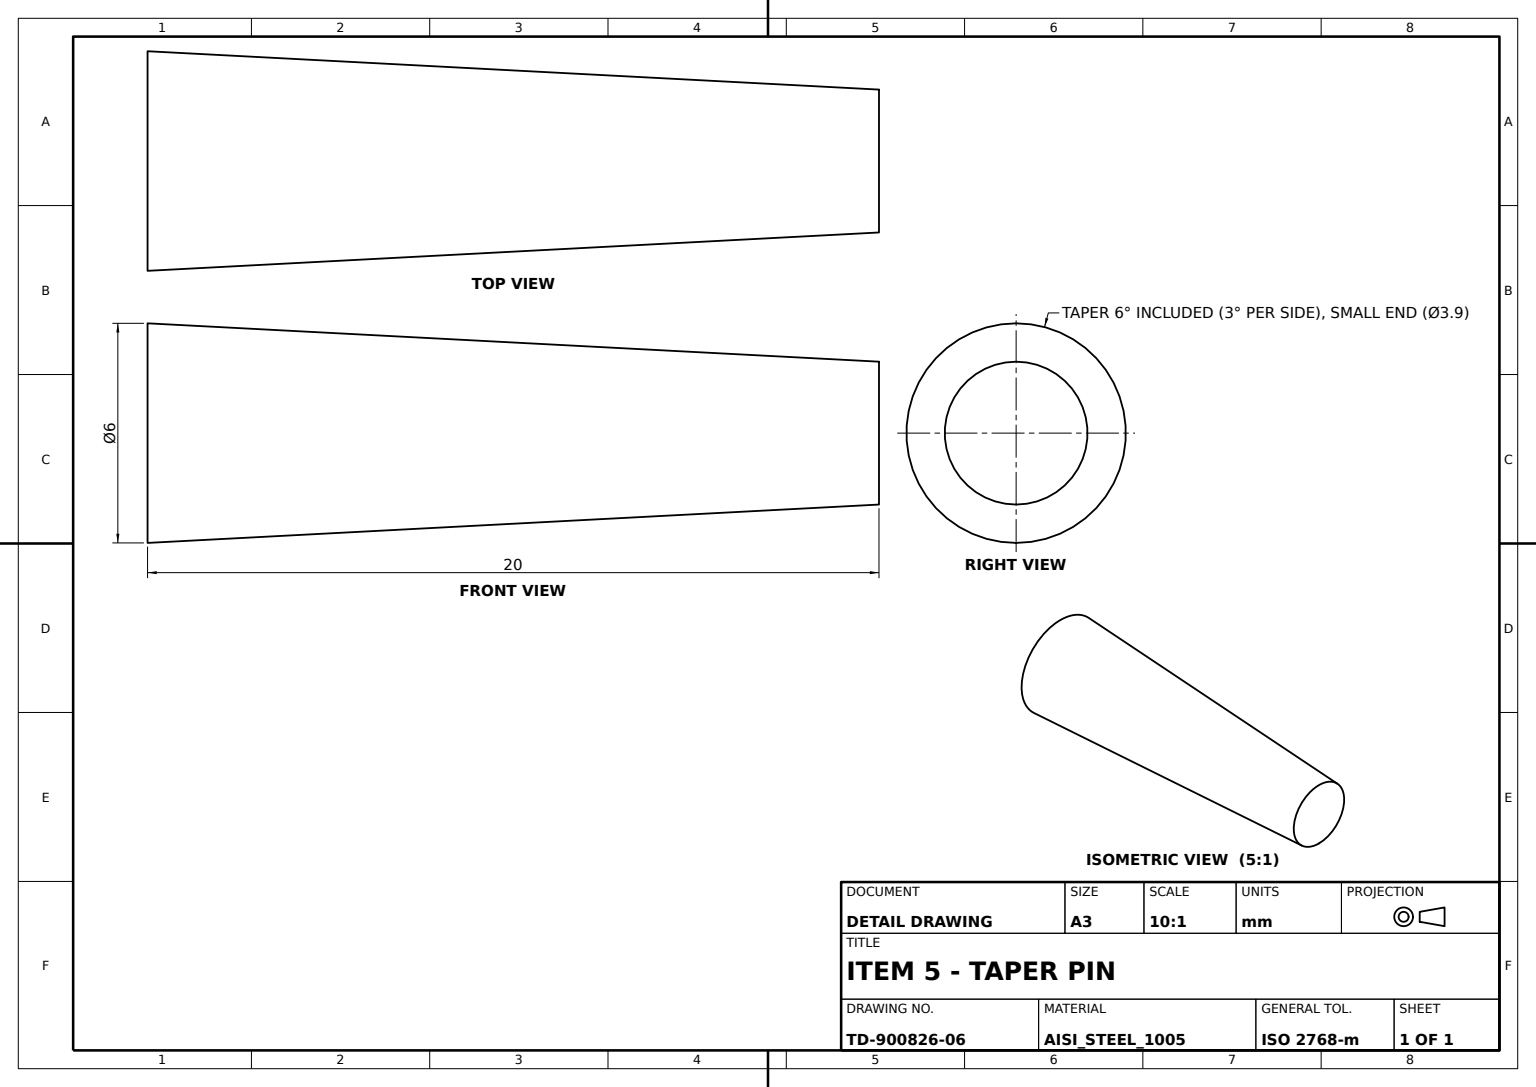
ISO-10303-21;
HEADER;
FILE_DESCRIPTION((''),'2;1');
FILE_NAME('','',(''),(''),'','','');
FILE_SCHEMA(('AUTOMOTIVE_DESIGN'));
ENDSEC;
DATA;
#1=APPLICATION_CONTEXT('');
#2=PRODUCT_CONTEXT('',#1,'mechanical');
#3=PRODUCT('','','',(#2));
#4=PRODUCT_DEFINITION_FORMATION('','',#3);
#5=PRODUCT_DEFINITION_CONTEXT('',#1,'design');
#6=PRODUCT_DEFINITION('','',#4,#5);
#7=PRODUCT_DEFINITION_SHAPE('','',#6);
#8=(LENGTH_UNIT()NAMED_UNIT(*)SI_UNIT(.MILLI.,.METRE.));
#9=(NAMED_UNIT(*)PLANE_ANGLE_UNIT()SI_UNIT($,.RADIAN.));
#10=(NAMED_UNIT(*)SI_UNIT($,.STERADIAN.)SOLID_ANGLE_UNIT());
#11=UNCERTAINTY_MEASURE_WITH_UNIT(LENGTH_MEASURE(0.005),#8,'distance_accuracy_value','');
#12=(GEOMETRIC_REPRESENTATION_CONTEXT(3)GLOBAL_UNCERTAINTY_ASSIGNED_CONTEXT((#11))GLOBAL_UNIT_ASSIGNED_CONTEXT((#8,#9,#10))REPRESENTATION_CONTEXT('',''));
#13=CARTESIAN_POINT('',(3.,0.,0.));
#14=VERTEX_POINT('',#13);
#15=CARTESIAN_POINT('',(0.,0.,0.));
#16=DIRECTION('',(0.,0.,1.));
#17=DIRECTION('',(1.,0.,0.));
#18=AXIS2_PLACEMENT_3D('',#15,#16,#17);
#19=CIRCLE('',#18,3.);
#20=EDGE_CURVE('',#14,#14,#19,.T.);
#21=ORIENTED_EDGE('',*,*,#20,.T.);
#22=EDGE_LOOP('',(#21));
#23=FACE_BOUND('',#22,.T.);
#24=CARTESIAN_POINT('',(1.951844,0.,20.));
#25=VERTEX_POINT('',#24);
#26=CARTESIAN_POINT('',(0.,0.,20.));
#27=AXIS2_PLACEMENT_3D('',#26,#16,#17);
#28=CIRCLE('',#27,1.951844);
#29=EDGE_CURVE('',#25,#25,#28,.T.);
#30=ORIENTED_EDGE('',*,*,#29,.F.);
#31=EDGE_LOOP('',(#30));
#32=FACE_BOUND('',#31,.T.);
#33=DIRECTION('',(0.,0.,-1.));
#34=AXIS2_PLACEMENT_3D('',#15,#33,#17);
#35=CONICAL_SURFACE('',#34,3.,0.052359878);
#36=ADVANCED_FACE('',(#23,#32),#35,.T.);
#37=ORIENTED_EDGE('',*,*,#20,.F.);
#38=EDGE_LOOP('',(#37));
#39=FACE_BOUND('',#38,.T.);
#40=PLANE('',#18);
#41=ADVANCED_FACE('',(#39),#40,.F.);
#42=ORIENTED_EDGE('',*,*,#29,.T.);
#43=EDGE_LOOP('',(#42));
#44=FACE_BOUND('',#43,.T.);
#45=PLANE('',#27);
#46=ADVANCED_FACE('',(#44),#45,.T.);
#47=CLOSED_SHELL('',(#36,#41,#46));
#48=MANIFOLD_SOLID_BREP('',#47);
#49=ADVANCED_BREP_SHAPE_REPRESENTATION('',(#48),#12);
#50=SHAPE_DEFINITION_REPRESENTATION(#7,#49);
ENDSEC;
END-ISO-10303-21;
